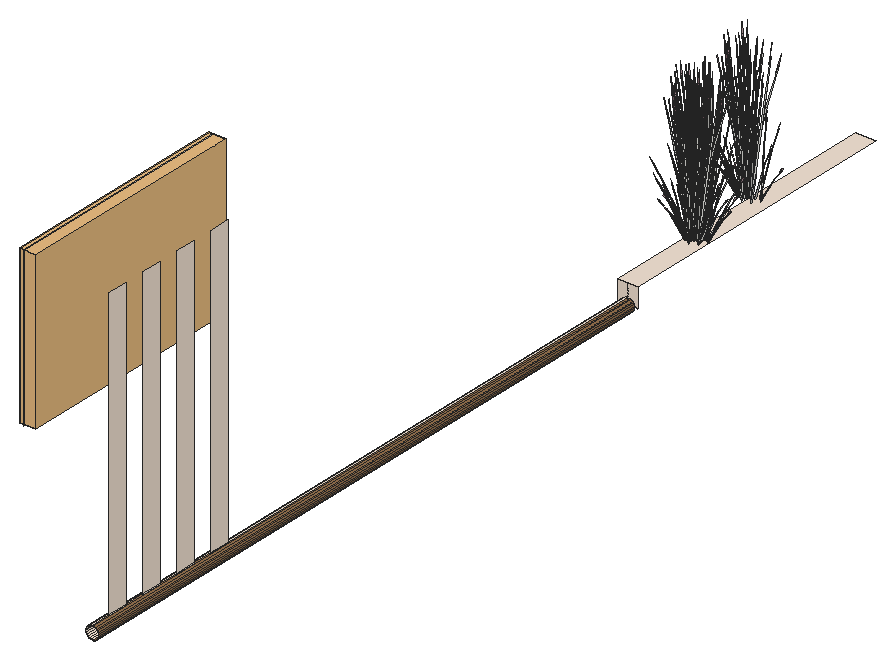
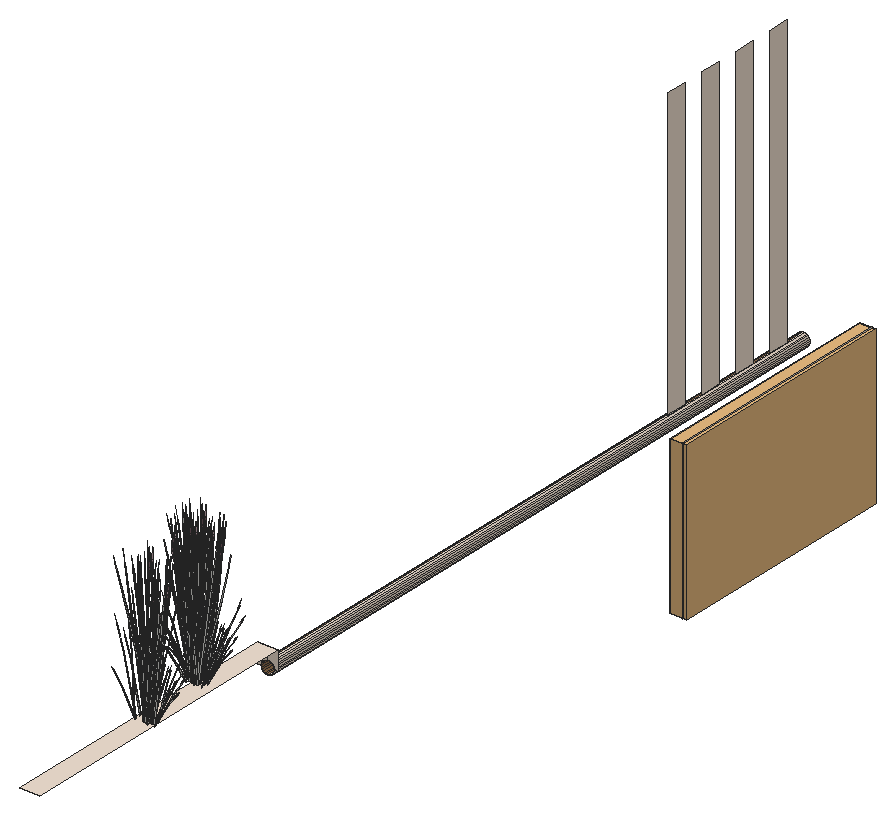
# SketchUp Ruby script. Lengths in inches.
U = 1.inch
M = Sketchup.active_model
def pt(a) = Geom::Point3d.new(a.map { |v| v * U })
def face(e, loops, mat)
  f = e.add_face(loops[0].map { |a| pt(a) })
  loops[1..].each { |l| e.add_face(l.map { |a| pt(a) }).erase! }
  f.material = f.back_material = mat if mat
  f
end
# faces: each face lists its corners as indices into pts; further lists are holes
def faces(e, pts, list, mat = nil) = list.each { |f| face(e, (f[0].is_a?(Array) ? f : [f]).map { |l| l.map { |i| pts[i] } }, mat) }
# xy, xz, yz: faces in a plane at the given z, y or x. An outline is a flat list of corners, or four numbers for a rectangle; further outlines are holes
def ring(l) = l.size == 4 ? [[l[0], l[1]], [l[2], l[1]], [l[2], l[3]], [l[0], l[3]]] : l.each_slice(2).to_a
def flat(e, list, mat, &to3) = list.each { |f| face(e, (f[0].is_a?(Array) ? f : [f]).map { |l| ring(l).map { |u, v| to3.(u, v) } }, mat) }
def xy(e, z, list, mat = nil) = flat(e, list, mat) { |x, y| [x, y, z] }
def xz(e, y, list, mat = nil) = flat(e, list, mat) { |x, z| [x, y, z] }
def yz(e, x, list, mat = nil) = flat(e, list, mat) { |y, z| [x, y, z] }
def lines(e, pts, list) = list.each { |a, b| e.add_line(pt(pts[a]), pt(pts[b])) }
# prism: a flat outline (further loops are holes) pulled along v
def prism(e, loops, v, mat = nil)
  f = face(e, loops, mat); d = Geom::Vector3d.new(v.map { |x| x * U })
  f.pushpull(f.normal.samedirection?(d) ? d.length : -d.length)
end
def box(e, o, s, mat = nil) = prism(e, [[o, [o[0] + s[0], o[1], o[2]], [o[0] + s[0], o[1] + s[1], o[2]], [o[0], o[1] + s[1], o[2]]]], [0, 0, s[2]], mat)
def at(x, y, z, deg = 0) = Geom::Transformation.translation(pt([x, y, z])) * Geom::Transformation.rotation(ORIGIN, Z_AXIS, deg.degrees)
def axes(o, x, y, z) = Geom::Transformation.new([*x, 0, *y, 0, *z, 0, *pt(o).to_a, 1])
def part(name) = M.definitions.add(name)
# library, detail: a bought-in or finely detailed component or shape, given as its bounding box
def library(name, o, s) = part(name).tap { |d| box(d.entities, o, s) }
def detail(e, o, s) = box(e.add_group.entities, o, s)
def put(e, d, t, mat = nil) = e.add_instance(d, t).tap { |i| i.material = mat if mat }
def group(e, t, mat = nil) = e.add_group.tap { |g| g.transformation = t; g.material = mat if mat }.entities
root = M.entities
M.materials.add("C01_Vanilla_Cream").color = [244, 228, 212]
M.materials.add("LightPink_Translucent").color = [144, 107, 117]
M.materials["LightPink_Translucent"].alpha = 0.75
M.materials.add("Wood_Floor_01_1K").color = [146, 111, 76]
c1 = library("Double casement window",[0,0,0],[5.02,56.42,60])
c2 = part("blade")
p = [[2.15,0.21,22],[0,0.17,0],[0.09,0.45,0],[2.18,0.31,22],[2.29,0.31,22],[0.38,0.45,0],
  [2.48,0.24,33],[2.49,0.24,33],[2.48,0.22,33]]
faces(c2.entities,p,[[0,1,2,3],[4,5,2,3],[6,3,4,7],[8,0,3,6]])
c3 = part("seeds")
p = [[0.3,-0.1,1.38],[-0.01,-0.03,1.59],[-0.01,-0.03,0.03],[0.14,-0.07,-0.07],[0.29,-0.03,3],[0.15,0.01,3.11]]
faces(c3.entities,p,[[0,1,2,3],[1,0,4,5]],"LightPink_Translucent")
c4 = part("blade with seeds")
put(c4.entities,c2,at(0,0,0))
put(c4.entities,c3,axes([2.4,0.25,30.99],[1.5799,-0.05474,1.17369],[-0.12525,1.92788,0.29478],[-0.07173,-0.02425,1.56792]))
xy(root,498,[[354,216,360,306.76]],"C01_Vanilla_Cream")
xz(root,216,[[354,492,355,492,355.07,492.52,355.27,493,355.59,493.41,356,493.73,356.48,493.93,357,494,357,498,354,498],[359,492,360,492,360,498,357,498,357,494,357.52,493.93,358,493.73,358.41,493.41,358.73,493,358.93,492.52]],"C01_Vanilla_Cream")
yz(root,288,[[[72,498,144,546],[109.5,501,141,543],[75,501,106.5,543]]],"C01_Vanilla_Cream")
yz(root,357,[[18.46,490,24.91,494],[31.37,490,37.83,494],[44.28,490,50.74,494],[57.2,490,63.65,494],[18.46,494,24.91,582],
  [31.37,494,37.83,582],[44.28,494,50.74,582],[57.2,494,63.65,582]],"C01_Vanilla_Cream")
p = [[356.48,216,490.07],[357,216,490],[357,63.65,490],[357,57.2,490],[357,50.74,490],[357,44.28,490],
  [357,37.83,490],[357,31.37,490],[357,24.91,490],[357,18.46,490],[357,12,490],[356.48,12,490.07],
  [357.52,216,490.07],[357.52,12,490.07],[356,216,490.27],[356,12,490.27],[358,216,490.27],[358,12,490.27],
  [355.59,216,490.59],[355.59,12,490.59],[358.41,216,490.59],[358.41,12,490.59],[355.27,216,491],[355.27,12,491],
  [358.73,216,491],[358.73,12,491],[355.07,216,491.48],[355.07,12,491.48],[358.93,216,491.48],[358.93,12,491.48],
  [355,216,492],[355,12,492],[359,216,492],[359,12,492],[355.07,216,492.52],[355.07,12,492.52],
  [358.93,216,492.52],[358.93,12,492.52],[355.27,216,493],[355.27,12,493],[358.73,216,493],[358.73,12,493],
  [355.59,216,493.41],[355.59,12,493.41],[358.41,216,493.41],[358.41,12,493.41],[356,216,493.73],[356,12,493.73],
  [358,216,493.73],[358,12,493.73],[356.48,216,493.93],[356.48,12,493.93],[357.52,216,493.93],[357.52,12,493.93],
  [357,216,494],[357,12,494],[357,18.46,494],[357,24.91,494],[357,31.37,494],[357,37.83,494],
  [357,44.28,494],[357,50.74,494],[357,57.2,494],[357,63.65,494]]
faces(root,p,[[0,1,2,3,4,5,6,7,8,9,10,11],[14,0,11,15],[18,14,15,19],[22,18,19,23],[26,22,23,27],[30,26,27,31],[34,30,31,35],[38,34,35,39],
  [42,38,39,43],[46,42,43,47],[50,46,47,51],[54,50,51,55,56,57,58,59,60,61,62,63]],"C01_Vanilla_Cream")
faces(root,p,[[1,12,13,10,9,8,7,6,5,4,3,2],[12,16,17,13],[16,20,21,17],[20,24,25,21],[24,28,29,25],[28,32,33,29],[32,36,37,33],[36,40,41,37],
  [40,44,45,41],[44,48,49,45],[48,52,53,49],[52,54,63,62,61,60,59,58,57,56,55,53]],"Wood_Floor_01_1K")
put(root,c1,axes([286.7,72.24,498.3],[1,0,0],[0,1.27666,0],[0,0,0.79394]))
put(root,c4,axes([358.96,239.09,499.94],[-0.15825,0.09972,1.07251],[-0.47395,-0.17454,-0.23066],[0.08785,-0.21706,0.45856]))
put(root,c4,axes([356.51,238.9,499.94],[-0.03371,0.16116,1.07251],[-0.49286,0.13491,-0.23066],[-0.11521,-0.20831,0.45856]))
put(root,c4,axes([357.78,238.55,499.12],[-0.09338,0.01775,1.32257],[-0.51641,-0.1998,-0.20205],[0.00867,-0.16666,0.22528]))
put(root,c4,axes([358.37,238.3,500.07],[0.07142,0.28728,0.86145],[-0.3962,-0.15911,0.63294],[0.04263,-0.1471,0.18974]))
put(root,c4,axes([356.34,238.64,500.07],[0.29042,0.17147,0.86145],[-0.42295,0.10307,0.63294],[-0.0905,-0.13178,0.18974]))
put(root,c4,axes([356.11,239.16,499.12],[-0.05393,0.0649,1.32257],[-0.545,0.13993,-0.20205],[-0.13166,-0.12729,0.22528]))
put(root,c4,axes([357.01,240.94,499.57],[-0.22864,-0.5052,-0.52377],[0.65862,-0.18195,-0.13747],[-0.02527,-0.17107,1.15612]))
put(root,c4,axes([360.0625,239.4,499.12],[-0.08333,-0.03881,1.32257],[-0.21404,-0.4336,-0.20205],[0.14439,-0.11767,0.22528]))
put(root,c4,axes([356.91,239.49,499.78],[-0.34808,-0.49367,0],[0.58235,-0.27531,-0.38706],[0.13264,-0.0627,1.22783]))
put(root,c4,axes([357.68,238.9,499.6],[-0.38473,0.28263,-0.02919],[-0.35252,-0.30954,-0.13237],[-0.02482,-0.08771,0.43661]))
put(root,c4,axes([355.66,240.87,499.51],[0,-0.49266,-0.37238],[0.62289,0,0],[0,-0.11221,1.18128]))
put(root,c4,axes([357.39,239.41,499.51],[0.52105,-0.24633,-0.37238],[0.31144,0.44171,0],[0.11867,-0.0561,1.18128]))
put(root,c4,axes([360.48,240.26,499.94],[-0.19889,-0.01459,1.07251],[-0.20376,-0.39145,-0.23066],[0.24434,-0.11074,0.45856]))
put(root,c4,axes([358.01,240.42,499.54],[0.375,-0.3703,-0.46765],[0.46584,0.33578,-0.12274],[0.15027,-0.09237,1.03225]))
put(root,c4,axes([360.71,239.55,500.07],[-0.18544,0.25079,0.86145],[-0.15939,-0.33694,0.63294],[0.15316,-0.08443,0.18974]))
put(root,c4,axes([357.35,241.07,499.66],[0.27012,-0.44393,-0.33554],[0.56127,0.21365,0.16149],[0,-0.10233,1.07733]))
put(root,c4,axes([357.6,240.85,500],[-0.06488,-0.56215,-0.21822],[0.6757,-0.03399,-0.37502],[0.11898,-0.07488,1.19781]))
put(root,c4,axes([355.92,240.88,499.52],[0.38863,-0.30738,-0.23233],[0.38863,0.30738,0.23233],[0,-0.09901,1.0423]))
put(root,c4,axes([355.77,239.41,499.6],[-0.1606,0.40228,-0.02919],[-0.4943,-0.12375,-0.13237],[-0.07505,-0.0658,0.43661]))
put(root,c4,axes([357.29,241.44,500],[-0.62699,-0.23507,-0.21822],[0.3019,-0.49615,-0.37502],[-0.0197,-0.12182,1.19781]))
put(root,c4,axes([355.5,241.25,499.78],[-0.69617,0,0],[0,-0.55062,-0.38706],[0,-0.12541,1.22783]))
put(root,c4,axes([355.62,240.26,499.94],[0.1087,0.13716,1.07251],[-0.25048,0.37284,-0.23066],[-0.25719,-0.08912,0.45856]))
put(root,c4,axes([357.51,239.61,499.52],[0.51941,0.1219,-0.23233],[-0.13078,0.42928,0.23233],[0.10471,-0.0495,1.0423]))
put(root,c4,axes([356.04,241.1,499.75],[-0.51786,0.4142,0.23067],[-0.51817,-0.40984,-0.27369],[-0.01808,-0.11762,1.23664]))
put(root,c4,axes([357.6875,241.29,499.82],[0.6273,0.23878,0.18048],[-0.3019,0.49615,0.37502],[0,-0.11437,1.20407]))
put(root,c4,axes([357.44,241.96,499.83],[0.14756,-0.58378,-0.17572],[0.69966,0.10176,0.38453],[-0.12225,-0.08062,1.1733]))
put(root,c4,axes([354.97,240.67,500.07],[0.35544,-0.03525,0.86145],[-0.22547,0.31061,0.63294],[-0.17565,-0.04659,0.18974]))
put(root,c4,axes([357.49,240.96,500.04],[-0.60457,0.03041,0.33554],[-0.05467,-0.50484,-0.16149],[0.10823,-0.05117,1.07733]))
put(root,c4,axes([355.92,241.33,499.86],[0,0.49266,0.37238],[-0.62289,0,0],[0,-0.11221,1.18128]))
put(root,c4,axes([359.48,239.61,499.78],[0.34808,-0.49367,0],[0.58235,0.27531,-0.38706],[0.13264,0.0627,1.22783]))
put(root,c4,axes([357.39,241.73,499.66],[-0.33445,-0.41351,-0.33554],[0.50659,-0.29119,0.16149],[-0.10823,-0.05117,1.07733]))
put(root,c4,axes([357.46,241.14,499.77],[0.24206,0.5509,0.34316],[-0.69162,0.19157,0.13466],[0.00845,-0.10123,1.19142]))
put(root,c4,axes([360.85,241.57,499.49],[-0.35858,0.05912,1.06187],[-0.05708,-0.47061,0.06078],[0.25115,-0.07123,0.60425]))
put(root,c4,axes([361.5,241.15,499.7],[-0.34516,-0.31503,-0.04866],[0.37803,-0.28865,-0.22062],[0.10711,-0.02032,0.72768]))
put(root,c4,axes([357.34,241.58,500.04],[-0.27012,0.44393,0.33554],[-0.56127,-0.21365,-0.16149],[0,-0.10233,1.07733]))
put(root,c4,axes([358.33,241.19,499.65],[0,-0.57005,0],[0.69617,0,0],[0,0,1.34592]))
put(root,c4,axes([359.18,239.87,499.86],[-0.52105,-0.24633,0.37238],[0.31144,-0.44171,0],[0.11867,0.0561,1.18128]))
put(root,c4,axes([357.09,241.89,499.54],[-0.57914,-0.08077,-0.46765],[0.12221,-0.49823,-0.12274],[-0.17283,-0.06037,1.03225]))
put(root,c4,axes([358,240.83,499.77],[-0.46162,0.4471,0.34316],[-0.54842,-0.39467,0.13466],[0.11129,-0.04462,1.19142]))
put(root,c4,axes([358.51,241.63,499.72],[-0.51786,-0.42404,-0.04598],[0.51817,-0.4243,0],[-0.01808,-0.01481,1.31678]))
put(root,c4,axes([357.2,240.09,499.86],[-0.16083,0.48962,0.13232],[-0.58854,-0.13856,0.26315],[0.10167,-0.00238,1.20305]))
put(root,c4,axes([356.96,240.49,499.2],[-0.548,0.19724,0.96696],[-0.17442,-0.56594,0.37572],[0.3365,0.00941,1.09981]))
put(root,c4,axes([358.43,240.64,499.96],[0.1074,-0.43968,0.1086],[0.52474,0.07632,-0.3101],[0.0955,0.04515,0.95058]))
put(root,c4,axes([357.52,241.68,499.77],[0.70367,0.1038,0.34316],[-0.1432,0.58624,0.13466],[-0.10283,-0.05661,1.19142]))
put(root,c4,axes([361.24,241.26,499.12],[-0.0291,-0.0748,1.32257],[0.20181,-0.43752,-0.20205],[0.20357,-0.00629,0.22528]))
put(root,c4,axes([355.23,241.18,499.12],[0.01412,0.07764,1.32257],[-0.28464,0.40547,-0.20205],[-0.20218,-0.02044,0.22528]))
put(root,c4,axes([358.21,240.75,500.04],[-0.33445,-0.41351,0.33554],[0.50659,-0.29119,-0.16149],[0.10823,0.05117,1.07733]))
put(root,c4,axes([356.48,242.64,499.52],[-0.13078,-0.42928,-0.23233],[0.51941,-0.1219,0.23233],[-0.10471,-0.0495,1.0423]))
put(root,c4,axes([357.15,242.62,499.86],[0.59825,-0.13076,0.13232],[0.14773,0.48663,0.26315],[-0.05336,-0.0709,1.20305]))
put(root,c4,axes([358.38,240.78,500],[0.56211,-0.32708,-0.21822],[0.3738,0.46216,-0.37502],[0.13869,0.04694,1.19781]))
put(root,c4,axes([356.33,242.83,499.51],[-0.52105,-0.24633,-0.37238],[0.31144,-0.44171,0],[-0.11867,-0.0561,1.18128]))
put(root,c4,axes([359.8,239.91,499.51],[0.52105,0.24633,-0.37238],[-0.31144,0.44171,0],[0.11867,0.0561,1.18128]))
put(root,c4,axes([358.81,241.32,499.65],[0.62289,0,0],[0,0.51004,0],[0,0,1.33805]))
put(root,c4,axes([357.75,241.96,500],[-0.56211,0.32708,-0.21822],[-0.3738,-0.46216,-0.37502],[-0.13869,-0.04694,1.19781]))
put(root,c4,axes([358.98,240.12,499.86],[-0.59825,0.13076,0.13232],[-0.14773,-0.48663,0.26315],[0.05336,0.0709,1.20305]))
put(root,c4,axes([359.65,240.1,499.52],[0.13078,0.42928,-0.23233],[-0.51941,0.1219,0.23233],[0.10471,0.0495,1.0423]))
put(root,c4,axes([358.61,241.06,499.79],[-0.70367,-0.1038,0.36899],[0.1432,-0.58624,0.1448],[0.10283,0.05661,1.2811]))
put(root,c4,axes([358.04,242.5,499.65],[-0.18165,-0.42474,0],[0.51872,-0.14874,0],[0,0,1.15778]))
put(root,c4,axes([357.7,242.1,499.96],[-0.1074,0.43968,0.1086],[-0.52474,-0.07632,-0.3101],[-0.0955,-0.04515,0.95058]))
put(root,c4,axes([358.72,242.45,499.64],[0.5845,-0.16716,-0.14398],[0.20539,0.48152,0.00006],[0.06452,-0.01848,1.30423]))
put(root,c4,axes([358.93,242.65,499.86],[0.16083,-0.48962,0.13232],[0.58854,0.13856,0.26315],[-0.10167,0.00238,1.20305]))
put(root,c4,axes([358.79,241.54,499.66],[0.38863,0.31822,0],[-0.38863,0.31822,0],[0,0,1.2695]))
put(root,c4,axes([359.85,241.4,499.86],[-0.43742,-0.35886,0.13232],[0.44081,-0.34807,0.26315],[-0.04831,0.07329,1.20305]))
put(root,c4,axes([359.04,240.86,499.54],[0.57914,0.08077,-0.46765],[-0.12221,0.49823,-0.12274],[0.17283,0.06037,1.03225]))
put(root,c4,axes([361.59,241.73,500.07],[-0.34399,0.08133,0.86145],[0.16192,-0.33614,0.63294],[0.18249,0.023,0.18974]))
put(root,c4,axes([357.92,242.7,499.65],[-0.56127,-0.22118,0],[0.27012,-0.45959,0],[0,0,1.2203]))
put(root,c4,axes([358.38,242.11,499.85],[-0.54364,-0.39653,-0.18894],[0.45745,-0.44527,0.41347],[-0.14639,0.04639,1.26162]))
put(root,c4,axes([356.95,242.87,499.86],[0.52105,0.24633,0.37238],[-0.31144,0.44171,0],[-0.11867,-0.0561,1.18128]))
put(root,c4,axes([358.79,241.16,500.04],[0.27012,-0.44393,0.33554],[0.56127,0.21365,-0.16149],[0,0.10233,1.07733]))
put(root,c4,axes([358.68,241.42,499.72],[0,0.56976,-0.04228],[-0.69617,0,0],[0,0.01791,1.34526]))
put(root,c4,axes([358.74,241.01,499.66],[0.33445,0.41351,-0.33554],[-0.50659,0.29119,0.16149],[0.10823,0.05117,1.07733]))
put(root,c4,axes([356.65,243.125,499.78],[-0.34808,0.49367,0],[-0.58235,-0.27531,-0.38706],[-0.13264,-0.0627,1.22783]))
put(root,c4,axes([360.21,241.41,499.86],[0,-0.49266,0.37238],[0.62289,0,0],[0,0.11221,1.18128]))
put(root,c4,axes([358.65,241.78,500.04],[0.60457,-0.03041,0.33554],[0.05467,0.50484,-0.16149],[-0.10823,0.05117,1.07733]))
put(root,c4,axes([359.02,241.26,499.96],[0.51872,-0.14368,0.1086],[0.18165,0.41027,-0.3101],[0,0.09029,0.95058]))
put(root,c4,axes([358.11,242.02,499.66],[-0.60457,0.03041,-0.33554],[-0.05467,-0.50484,0.16149],[-0.10823,0.05117,1.07733]))
put(root,c4,axes([360.95,242.26,499.94],[-0.13408,-0.12117,1.07251],[0.17446,-0.40083,-0.23066],[0.27128,0.0543,0.45856]))
put(root,c4,axes([358.55,242.71,499.65],[0.56127,0.22118,0],[-0.27012,0.45959,0],[0,0,1.31215]))
put(root,c4,axes([358.78,243.19,499.64],[-0.34375,-0.4954,-0.03857],[0.58235,-0.27531,0.38706],[-0.1435,0.04717,1.22723]))
put(root,c4,axes([358.66,242,499.96],[0.41131,0.296,0.1086],[-0.34309,0.33395,-0.3101],[-0.0955,0.04515,0.95058]))
put(root,c4,axes([359.09,242.91,499.86],[0.52105,-0.24633,0.37238],[0.31144,0.44171,0],[-0.11867,0.0561,1.18128]))
put(root,c4,axes([358.35,242.52,499.72],[0.24206,0.56598,-0.04509],[-0.69162,0.19832,0],[0.00845,0.01976,1.2913]))
put(root,c4,axes([358.62,243.13,499.52],[-0.51941,-0.1219,-0.23233],[0.13078,-0.42928,0.23233],[-0.10471,0.0495,1.0423]))
put(root,c4,axes([354.87,242.26,499.94],[0.19348,0.04044,1.07251],[0.1247,0.41309,-0.23066],[-0.26282,0.07733,0.45856]))
put(root,c4,axes([360.63,241.49,499.78],[0.69617,0,0],[0,0.55062,-0.38706],[0,0.12541,1.22783]))
put(root,c4,axes([360.35,241.78,499.65],[-0.69582,-0.00394,-0.03732],[0,-0.55062,0.37457],[-0.02187,0.12535,1.18764]))
put(root,c4,axes([358.84,241.3,500],[0.62699,0.23507,-0.21822],[-0.3019,0.49615,-0.37502],[0.0197,0.12182,1.19781]))
put(root,c4,axes([354.47,243.125,500.07],[0.23202,-0.22328,0.86145],[0.09155,0.35348,0.63294],[-0.16768,0.06329,0.18974]))
put(root,c4,axes([360.21,241.86,499.52],[-0.38863,0.30738,-0.23233],[-0.38863,-0.30738,0.23233],[0,0.09901,1.0423]))
put(root,c4,axes([358.53,241.89,500],[0.06488,0.56215,-0.21822],[-0.6757,0.03399,-0.37502],[-0.11898,0.07488,1.19781]))
put(root,c4,axes([358.78,241.67,499.66],[-0.27012,0.44393,-0.33554],[-0.56127,-0.21365,0.16149],[0,0.10233,1.07733]))
put(root,c4,axes([358.125,242.32,499.54],[-0.375,0.3703,-0.46765],[-0.46584,-0.33578,-0.12274],[-0.15027,0.09237,1.03225]))
put(root,c4,axes([358.79,242.94,499.75],[0.697,0.16013,0.23067],[-0.17437,0.57237,-0.27369],[-0.11536,0.07164,1.23664]))
put(root,c4,axes([358.74,243.33,499.51],[-0.52105,0.24633,-0.37238],[-0.31144,-0.44171,0],[-0.11867,0.0561,1.18128]))
put(root,c4,axes([360.47,241.87,499.51],[0,0.49266,-0.37238],[-0.62289,0,0],[0,0.11221,1.18128]))
put(root,c4,axes([359.68,242.89,500.07],[-0.31347,-0.14166,0.86145],[0.40476,-0.14393,0.63294],[0.10917,0.12192,0.18974]))
put(root,c4,axes([359.22,243.25,499.78],[0.34808,0.49367,0],[-0.58235,0.27531,-0.38706],[-0.13264,0.0627,1.22783]))
put(root,c4,axes([359.77,243.42,499.12],[0.04056,-0.07113,1.32257],[0.51066,-0.20948,-0.20205],[0.15482,0.10842,0.22528]))
put(root,c4,axes([359.1,241.8,499.57],[0.20414,0.45107,-0.51909],[-0.58805,0.16245,-0.13624],[0.02256,0.15274,1.1458]))
put(root,c4,axes([355.08,243.36,499.12],[0.07468,0.04922,1.32257],[0.12663,0.45605,-0.20205],[-0.16551,0.09725,0.22528]))
put(root,c4,axes([359.73,243.54,500],[-0.35702,-0.01545,0.78795],[0.23577,-0.32816,0.43504],[0.14104,0.11659,0.61808]))
put(root,c4,axes([358.57,242.74,499.94],[0.00982,-0.16331,1.07251],[0.4695,-0.18242,-0.23066],[0.14493,0.19547,0.45856]))
put(root,c4,axes([356.4375,244.1,500.07],[-0.01441,-0.29294,0.86145],[0.36003,0.20894,0.63294],[-0.07081,0.13963,0.18974]))
put(root,c4,axes([357.38,243.4,499.12],[0.0901,-0.02681,1.32257],[0.54199,0.14755,-0.20205],[0.01585,0.1663,0.22528]))
put(root,c4,axes([356.14,243.47,500.12],[0.50577,-0.08724,0.04881],[0.11627,0.35148,-0.64728],[-0.03206,0.17792,0.5802]))
put(root,c4,axes([356.02,243.84,499.94],[0.17569,-0.07772,1.07251],[0.43377,0.23434,-0.23066],[-0.12911,0.20277,0.45856]))
put(root,c4,axes([355.92,263.06,499.94],[-0.15825,0.09972,1.07251],[-0.47395,-0.17454,-0.23066],[0.08785,-0.21706,0.45856]))
put(root,c4,axes([353.47,262.87,499.94],[-0.03371,0.16116,1.07251],[-0.49286,0.13491,-0.23066],[-0.11521,-0.20831,0.45856]))
put(root,c4,axes([354.74,262.52,499.12],[-0.09338,0.01775,1.32257],[-0.51641,-0.1998,-0.20205],[0.00867,-0.16666,0.22528]))
put(root,c4,axes([353.3,262.61,500.07],[0.29042,0.17147,0.86145],[-0.42295,0.10307,0.63294],[-0.0905,-0.13178,0.18974]))
put(root,c4,axes([353.07,263.125,499.12],[-0.05393,0.0649,1.32257],[-0.545,0.13993,-0.20205],[-0.13166,-0.12729,0.22528]))
put(root,c4,axes([353.97,264.91,499.57],[-0.22864,-0.5052,-0.52377],[0.65862,-0.18195,-0.13747],[-0.02527,-0.17107,1.15612]))
put(root,c4,axes([357.02,263.37,499.12],[-0.08333,-0.03881,1.32257],[-0.21404,-0.4336,-0.20205],[0.14439,-0.11767,0.22528]))
put(root,c4,axes([353.88,263.46,499.78],[-0.34808,-0.49367,0],[0.58235,-0.27531,-0.38706],[0.13264,-0.0627,1.22783]))
put(root,c4,axes([354.64,262.86,499.6],[-0.38473,0.28263,-0.02919],[-0.35252,-0.30954,-0.13237],[-0.02482,-0.08771,0.43661]))
put(root,c4,axes([352.62,264.84,499.51],[0,-0.49266,-0.37238],[0.62289,0,0],[0,-0.11221,1.18128]))
put(root,c4,axes([354.35,263.38,499.51],[0.52105,-0.24633,-0.37238],[0.31144,0.44171,0],[0.11867,-0.0561,1.18128]))
put(root,c4,axes([357.44,264.23,499.94],[-0.19889,-0.01459,1.07251],[-0.20376,-0.39145,-0.23066],[0.24434,-0.11074,0.45856]))
put(root,c4,axes([354.97,264.39,499.54],[0.375,-0.3703,-0.46765],[0.46584,0.33578,-0.12274],[0.15027,-0.09237,1.03225]))
put(root,c4,axes([354.31,265.04,499.66],[0.27012,-0.44393,-0.33554],[0.56127,0.21365,0.16149],[0,-0.10233,1.07733]))
put(root,c4,axes([354.5625,264.82,500],[-0.06488,-0.56215,-0.21822],[0.6757,-0.03399,-0.37502],[0.11898,-0.07488,1.19781]))
put(root,c4,axes([352.89,264.85,499.52],[0.38863,-0.30738,-0.23233],[0.38863,0.30738,0.23233],[0,-0.09901,1.0423]))
put(root,c4,axes([352.73,263.375,499.6],[-0.1606,0.40228,-0.02919],[-0.4943,-0.12375,-0.13237],[-0.07505,-0.0658,0.43661]))
put(root,c4,axes([354.25,265.41,500],[-0.62699,-0.23507,-0.21822],[0.3019,-0.49615,-0.37502],[-0.0197,-0.12182,1.19781]))
put(root,c4,axes([352.46,265.21,499.78],[-0.69617,0,0],[0,-0.55062,-0.38706],[0,-0.12541,1.22783]))
put(root,c4,axes([352.58,264.23,499.94],[0.1087,0.13716,1.07251],[-0.25048,0.37284,-0.23066],[-0.25719,-0.08912,0.45856]))
put(root,c4,axes([354.47,263.58,499.52],[0.51941,0.1219,-0.23233],[-0.13078,0.42928,0.23233],[0.10471,-0.0495,1.0423]))
put(root,c4,axes([353,265.07,499.75],[-0.51786,0.4142,0.23067],[-0.51817,-0.40984,-0.27369],[-0.01808,-0.11762,1.23664]))
put(root,c4,axes([354.65,265.26,499.82],[0.6273,0.23878,0.18048],[-0.3019,0.49615,0.37502],[0,-0.11437,1.20407]))
put(root,c4,axes([354.41,265.93,499.83],[0.14756,-0.58378,-0.17572],[0.69966,0.10176,0.38453],[-0.12225,-0.08062,1.1733]))
put(root,c4,axes([351.9375,264.64,500.07],[0.35544,-0.03525,0.86145],[-0.22547,0.31061,0.63294],[-0.17565,-0.04659,0.18974]))
put(root,c4,axes([354.45,264.93,500.04],[-0.60457,0.03041,0.33554],[-0.05467,-0.50484,-0.16149],[0.10823,-0.05117,1.07733]))
put(root,c4,axes([352.89,265.3,499.86],[0,0.49266,0.37238],[-0.62289,0,0],[0,-0.11221,1.18128]))
put(root,c4,axes([356.44,263.58,499.78],[0.34808,-0.49367,0],[0.58235,0.27531,-0.38706],[0.13264,0.0627,1.22783]))
put(root,c4,axes([354.36,265.69,499.66],[-0.33445,-0.41351,-0.33554],[0.50659,-0.29119,0.16149],[-0.10823,-0.05117,1.07733]))
put(root,c4,axes([354.43,265.11,499.77],[0.24206,0.5509,0.34316],[-0.69162,0.19157,0.13466],[0.00845,-0.10123,1.19142]))
put(root,c4,axes([357.8125,265.53,499.49],[-0.35858,0.05912,1.06187],[-0.05708,-0.47061,0.06078],[0.25115,-0.07123,0.60425]))
put(root,c4,axes([358.46,265.12,499.7],[-0.34516,-0.31503,-0.04866],[0.37803,-0.28865,-0.22062],[0.10711,-0.02032,0.72768]))
put(root,c4,axes([354.3,265.54,500.04],[-0.27012,0.44393,0.33554],[-0.56127,-0.21365,-0.16149],[0,-0.10233,1.07733]))
put(root,c4,axes([355.3,265.16,499.65],[0,-0.57005,0],[0.69617,0,0],[0,0,1.34592]))
put(root,c4,axes([356.14,263.84,499.86],[-0.52105,-0.24633,0.37238],[0.31144,-0.44171,0],[0.11867,0.0561,1.18128]))
put(root,c4,axes([354.06,265.85,499.54],[-0.57914,-0.08077,-0.46765],[0.12221,-0.49823,-0.12274],[-0.17283,-0.06037,1.03225]))
put(root,c4,axes([354.97,264.8,499.77],[-0.46162,0.4471,0.34316],[-0.54842,-0.39467,0.13466],[0.11129,-0.04462,1.19142]))
put(root,c4,axes([355.47,265.6,499.72],[-0.51786,-0.42404,-0.04598],[0.51817,-0.4243,0],[-0.01808,-0.01481,1.31678]))
put(root,c4,axes([354.17,264.0625,499.86],[-0.16083,0.48962,0.13232],[-0.58854,-0.13856,0.26315],[0.10167,-0.00238,1.20305]))
put(root,c4,axes([353.92,264.46,499.2],[-0.548,0.19724,0.96696],[-0.17442,-0.56594,0.37572],[0.3365,0.00941,1.09981]))
put(root,c4,axes([355.39,264.61,499.96],[0.1074,-0.43968,0.1086],[0.52474,0.07632,-0.3101],[0.0955,0.04515,0.95058]))
put(root,c4,axes([354.49,265.65,499.77],[0.70367,0.1038,0.34316],[-0.1432,0.58624,0.13466],[-0.10283,-0.05661,1.19142]))
put(root,c4,axes([358.2,265.22,499.12],[-0.0291,-0.0748,1.32257],[0.20181,-0.43752,-0.20205],[0.20357,-0.00629,0.22528]))
put(root,c4,axes([352.19,265.15,499.12],[0.01412,0.07764,1.32257],[-0.28464,0.40547,-0.20205],[-0.20218,-0.02044,0.22528]))
put(root,c4,axes([355.17,264.72,500.04],[-0.33445,-0.41351,0.33554],[0.50659,-0.29119,-0.16149],[0.10823,0.05117,1.07733]))
